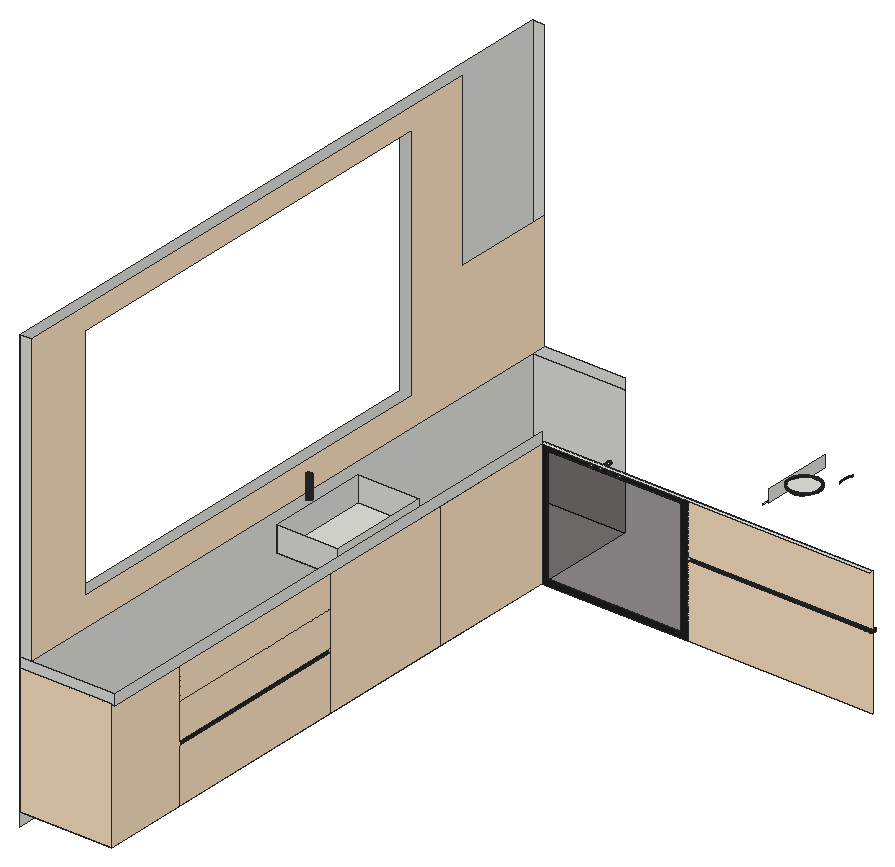
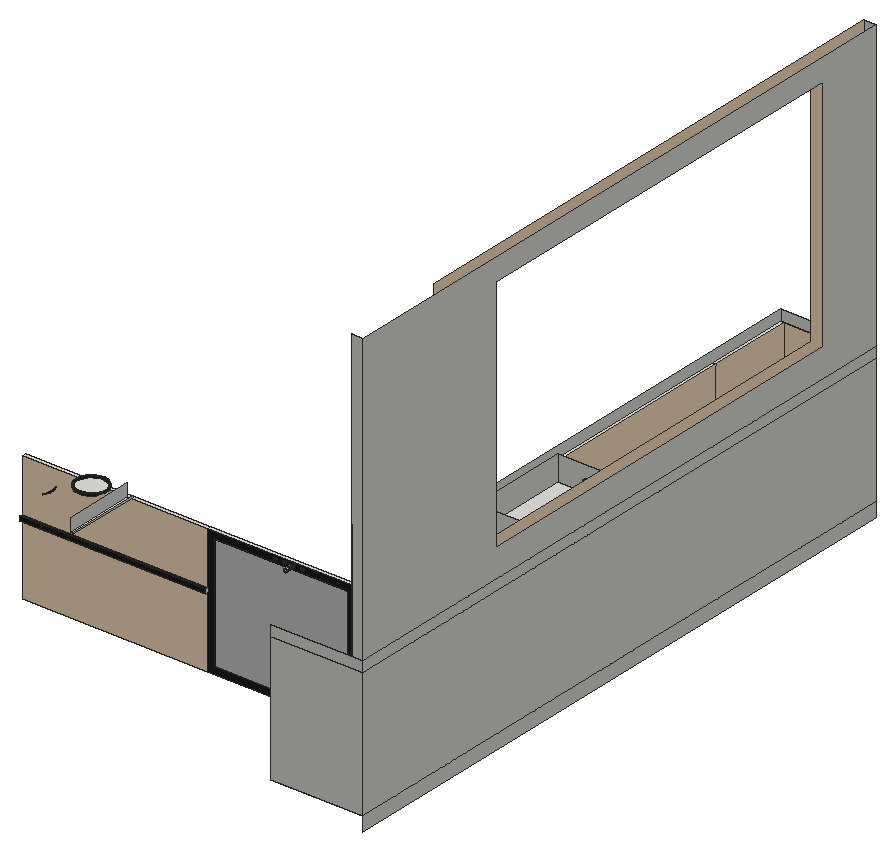
# SketchUp Ruby script. Lengths in inches.
U = 1.inch
M = Sketchup.active_model
def pt(a) = Geom::Point3d.new(a.map { |v| v * U })
def face(e, loops, mat)
  f = e.add_face(loops[0].map { |a| pt(a) })
  loops[1..].each { |l| e.add_face(l.map { |a| pt(a) }).erase! }
  f.material = f.back_material = mat if mat
  f
end
# faces: each face lists its corners as indices into pts; further lists are holes
def faces(e, pts, list, mat = nil) = list.each { |f| face(e, (f[0].is_a?(Array) ? f : [f]).map { |l| l.map { |i| pts[i] } }, mat) }
# xy, xz, yz: faces in a plane at the given z, y or x. An outline is a flat list of corners, or four numbers for a rectangle; further outlines are holes
def ring(l) = l.size == 4 ? [[l[0], l[1]], [l[2], l[1]], [l[2], l[3]], [l[0], l[3]]] : l.each_slice(2).to_a
def flat(e, list, mat, &to3) = list.each { |f| face(e, (f[0].is_a?(Array) ? f : [f]).map { |l| ring(l).map { |u, v| to3.(u, v) } }, mat) }
def xy(e, z, list, mat = nil) = flat(e, list, mat) { |x, y| [x, y, z] }
def xz(e, y, list, mat = nil) = flat(e, list, mat) { |x, z| [x, y, z] }
def yz(e, x, list, mat = nil) = flat(e, list, mat) { |y, z| [x, y, z] }
def lines(e, pts, list) = list.each { |a, b| e.add_line(pt(pts[a]), pt(pts[b])) }
# prism: a flat outline (further loops are holes) pulled along v
def prism(e, loops, v, mat = nil)
  f = face(e, loops, mat); d = Geom::Vector3d.new(v.map { |x| x * U })
  f.pushpull(f.normal.samedirection?(d) ? d.length : -d.length)
end
def box(e, o, s, mat = nil) = prism(e, [[o, [o[0] + s[0], o[1], o[2]], [o[0] + s[0], o[1] + s[1], o[2]], [o[0], o[1] + s[1], o[2]]]], [0, 0, s[2]], mat)
def at(x, y, z, deg = 0) = Geom::Transformation.translation(pt([x, y, z])) * Geom::Transformation.rotation(ORIGIN, Z_AXIS, deg.degrees)
def axes(o, x, y, z) = Geom::Transformation.new([*x, 0, *y, 0, *z, 0, *pt(o).to_a, 1])
def part(name) = M.definitions.add(name)
# library, detail: a bought-in or finely detailed component or shape, given as its bounding box
def library(name, o, s) = part(name).tap { |d| box(d.entities, o, s) }
def detail(e, o, s) = box(e.add_group.entities, o, s)
def put(e, d, t, mat = nil) = e.add_instance(d, t).tap { |i| i.material = mat if mat }
def group(e, t, mat = nil) = e.add_group.tap { |g| g.transformation = t; g.material = mat if mat }.entities
root = M.entities
M.materials.add("[0012_Bisque]").color = [255, 228, 196]
M.materials.add("[Color M00]").color = [255, 255, 255]
M.materials.add("[Color M08]").color = [30, 30, 30]
M.materials.add("[Translucent Glass Dark Green]").color = [11, 0, 5]
M.materials["[Translucent Glass Dark Green]"].alpha = 0.5
xy(root,0,[[0,2.74,25.8125,182.74]])
xy(root,15.1875,[[25.0625,26.49,25.8125,79.68]],"[Color M08]")
xy(root,16.375,[[25.0625,26.49,25.8125,79.68]],"[Color M08]")
xy(root,20.125,[[66.75,153.74,118.875,154.62]],"[Color M08]")
xy(root,21.25,[[66.75,153.74,118.875,154.62]],"[Color M08]")
xy(root,32.0625,[[7.17,83.87,24.36,112.5]])
xy(root,36,[[25.8125,2.74,26.71,26.49],[25.8125,26.49,26.71,79.68],[25.8125,79.68,26.71,118],[25.8125,118,26.71,153.74],[26.71,152.62,66.75,153.74],
  [66.75,152.62,118.875,153.74]])
xy(root,39,[[0,2.74,3.25,182.74],[5.34,96.75,5.13,96.8,4.95,96.91,4.79,97.05,4.68,97.23,4.62,97.4375,4.62,97.65,4.67,97.85,4.77,98.04,4.91,98.19,5.1,98.31,5.3,98.36,5.51,98.37,5.72,98.32,5.9,98.22,6.06,98.07,6.17,97.89,6.23,97.6875,6.23,97.48,6.18,97.27,6.08,97.08,5.93,96.93,5.75,96.82,5.55,96.76]])
xy(root,39.4375,[[84.98,158.42,85.73,178.23]])
xy(root,42.875,[[90.73,160.4,91.76,160.46,92.74,160.79,93.6,161.37,94.28,162.14,94.74,163.07,94.94,164.08,94.875,165.11,94.54,166.09,93.97,166.95,93.19,167.63,92.27,168.09,91.26,168.29,90.22,168.23,89.25,167.9,88.39,167.32,87.7,166.55,87.25,165.62,87.04,164.61,87.11,163.58,87.44,162.6,88.01,161.74,88.79,161.06,89.71,160.6]])
xy(root,42.875,[[[90.7,160.04,89.6,160.26,88.59,160.76,87.74,161.51,87.12,162.44,86.76,163.51,86.6875,164.63,86.91,165.74,87.41,166.75,88.15,167.59,89.09,168.22,90.16,168.58,91.28,168.65,92.38,168.43,93.39,167.93,94.24,167.18,94.86,166.25,95.22,165.18,95.29,164.06,95.07,162.95,94.57,161.94,93.83,161.1,92.89,160.47,91.83,160.11],[90.73,160.4,91.76,160.46,92.74,160.79,93.6,161.37,94.28,162.14,94.74,163.07,94.94,164.08,94.875,165.11,94.54,166.09,93.97,166.95,93.19,167.63,92.27,168.09,91.26,168.29,90.22,168.23,89.25,167.9,88.39,167.32,87.7,166.55,87.25,165.62,87.04,164.61,87.11,163.58,87.44,162.6,88.01,161.74,88.79,161.06,89.71,160.6]]],"[Color M08]")
xy(root,43.3125,[[[90.7,160.04,91.83,160.11,92.89,160.47,93.83,161.1,94.57,161.94,95.07,162.95,95.29,164.06,95.22,165.18,94.86,166.25,94.24,167.18,93.39,167.93,92.38,168.43,91.28,168.65,90.16,168.58,89.09,168.22,88.15,167.59,87.41,166.75,86.91,165.74,86.6875,164.63,86.76,163.51,87.12,162.44,87.74,161.51,88.59,160.76,89.6,160.26],[90.73,160.4,89.71,160.6,88.79,161.06,88.01,161.74,87.44,162.6,87.11,163.58,87.04,164.61,87.25,165.62,87.7,166.55,88.39,167.32,89.25,167.9,90.22,168.23,91.26,168.29,92.27,168.09,93.19,167.63,93.97,166.95,94.54,166.09,94.875,165.11,94.94,164.08,94.74,163.07,94.28,162.14,93.6,161.37,92.74,160.79,91.76,160.46]]],"[Color M08]")
xz(root,2.74,[[0,36,26.71,39],[0,39,3.25,120]])
xz(root,2.74,[[0,0,25.8125,36]],"[0012_Bisque]")
xz(root,26.49,[[25.0625,15.1875,25.8125,16.375]])
xz(root,79.68,[[25.0625,15.1875,25.8125,16.375]])
xz(root,83.87,[[7.17,32.0625,24.36,39]])
xz(root,112.5,[[7.17,32.0625,24.36,39]])
xz(root,153.24,[[40.09,34.75,40.2,34.76,40.31,34.81,40.4,34.88,40.47,34.97,40.51,35.07,40.53,35.1875,40.51,35.3,40.47,35.41,40.4,35.5,40.31,35.57,40.2,35.61,40.09,35.625,39.98,35.61,39.87,35.57,39.78,35.5,39.71,35.41,39.67,35.3,39.65,35.1875,39.67,35.07,39.71,34.97,39.78,34.88,39.87,34.81,39.98,34.76],[42.72,34.75,42.83,34.76,42.94,34.81,43.03,34.88,43.1,34.97,43.14,35.07,43.15,35.1875,43.14,35.3,43.1,35.41,43.03,35.5,42.94,35.57,42.83,35.61,42.72,35.625,42.6,35.61,42.5,35.57,42.41,35.5,42.34,35.41,42.29,35.3,42.28,35.1875,42.29,35.07,42.34,34.97,42.41,34.88,42.5,34.81,42.6,34.76],[45.28,34.75,45.39,34.76,45.5,34.81,45.59,34.88,45.66,34.97,45.7,35.07,45.72,35.1875,45.7,35.3,45.66,35.41,45.59,35.5,45.5,35.57,45.39,35.61,45.28,35.625,45.17,35.61,45.06,35.57,44.97,35.5,44.9,35.41,44.86,35.3,44.84,35.1875,44.86,35.07,44.9,34.97,44.97,34.88,45.06,34.81,45.17,34.76],[47.97,34.75,48.08,34.76,48.19,34.81,48.28,34.88,48.35,34.97,48.39,35.07,48.4,35.1875,48.39,35.3,48.35,35.41,48.28,35.5,48.19,35.57,48.08,35.61,47.97,35.625,47.85,35.61,47.75,35.57,47.66,35.5,47.59,35.41,47.54,35.3,47.53,35.1875,47.54,35.07,47.59,34.97,47.66,34.88,47.75,34.81,47.85,34.76]],"[Color M00]")
xz(root,153.74,[[66.75,0,118.875,20.125],[66.75,21.25,118.875,36]],"[0012_Bisque]")
xz(root,153.74,[[40.09,34.75,39.98,34.76,39.87,34.81,39.78,34.88,39.71,34.97,39.67,35.07,39.65,35.1875,39.67,35.3,39.71,35.41,39.78,35.5,39.87,35.57,39.98,35.61,40.09,35.625,40.2,35.61,40.31,35.57,40.4,35.5,40.47,35.41,40.51,35.3,40.53,35.1875,40.51,35.07,40.47,34.97,40.4,34.88,40.31,34.81,40.2,34.76],[42.72,34.75,42.6,34.76,42.5,34.81,42.41,34.88,42.34,34.97,42.29,35.07,42.28,35.1875,42.29,35.3,42.34,35.41,42.41,35.5,42.5,35.57,42.6,35.61,42.72,35.625,42.83,35.61,42.94,35.57,43.03,35.5,43.1,35.41,43.14,35.3,43.15,35.1875,43.14,35.07,43.1,34.97,43.03,34.88,42.94,34.81,42.83,34.76],[45.28,34.75,45.17,34.76,45.06,34.81,44.97,34.88,44.9,34.97,44.86,35.07,44.84,35.1875,44.86,35.3,44.9,35.41,44.97,35.5,45.06,35.57,45.17,35.61,45.28,35.625,45.39,35.61,45.5,35.57,45.59,35.5,45.66,35.41,45.7,35.3,45.72,35.1875,45.7,35.07,45.66,34.97,45.59,34.88,45.5,34.81,45.39,34.76],[47.97,34.75,47.85,34.76,47.75,34.81,47.66,34.88,47.59,34.97,47.54,35.07,47.53,35.1875,47.54,35.3,47.59,35.41,47.66,35.5,47.75,35.57,47.85,35.61,47.97,35.625,48.08,35.61,48.19,35.57,48.28,35.5,48.35,35.41,48.39,35.3,48.4,35.1875,48.39,35.07,48.35,34.97,48.28,34.88,48.19,34.81,48.08,34.76]],"[Color M00]")
xz(root,153.74,[[[25.8125,0,66.75,36],[27.6,1.79,64.96,34.21],[40.09,34.75,39.98,34.76,39.87,34.81,39.78,34.88,39.71,34.97,39.67,35.07,39.65,35.1875,39.67,35.3,39.71,35.41,39.78,35.5,39.87,35.57,39.98,35.61,40.09,35.625,40.2,35.61,40.31,35.57,40.4,35.5,40.47,35.41,40.51,35.3,40.53,35.1875,40.51,35.07,40.47,34.97,40.4,34.88,40.31,34.81,40.2,34.76],[42.72,34.75,42.6,34.76,42.5,34.81,42.41,34.88,42.34,34.97,42.29,35.07,42.28,35.1875,42.29,35.3,42.34,35.41,42.41,35.5,42.5,35.57,42.6,35.61,42.72,35.625,42.83,35.61,42.94,35.57,43.03,35.5,43.1,35.41,43.14,35.3,43.15,35.1875,43.14,35.07,43.1,34.97,43.03,34.88,42.94,34.81,42.83,34.76],[45.28,34.75,45.17,34.76,45.06,34.81,44.97,34.88,44.9,34.97,44.86,35.07,44.84,35.1875,44.86,35.3,44.9,35.41,44.97,35.5,45.06,35.57,45.17,35.61,45.28,35.625,45.39,35.61,45.5,35.57,45.59,35.5,45.66,35.41,45.7,35.3,45.72,35.1875,45.7,35.07,45.66,34.97,45.59,34.88,45.5,34.81,45.39,34.76],[47.97,34.75,47.85,34.76,47.75,34.81,47.66,34.88,47.59,34.97,47.54,35.07,47.53,35.1875,47.54,35.3,47.59,35.41,47.66,35.5,47.75,35.57,47.85,35.61,47.97,35.625,48.08,35.61,48.19,35.57,48.28,35.5,48.35,35.41,48.39,35.3,48.4,35.1875,48.39,35.07,48.35,34.97,48.28,34.88,48.19,34.81,48.08,34.76]]],"[Color M08]")
xz(root,153.74,[[27.6,1.79,64.96,34.21]],"[Translucent Glass Dark Green]")
xz(root,154.62,[[66.75,20.125,118.875,21.25]],"[Color M08]")
xz(root,156.55,[[42.72,34.75,42.6,34.76,42.5,34.81,42.41,34.88,42.34,34.97,42.29,35.07,42.28,35.1875,42.29,35.3,42.34,35.41,42.41,35.5,42.5,35.57,42.6,35.61,42.72,35.625,42.83,35.61,42.94,35.57,43.03,35.5,43.1,35.41,43.14,35.3,43.15,35.1875,43.14,35.07,43.1,34.97,43.03,34.88,42.94,34.81,42.83,34.76]],"[Color M00]")
xz(root,182.74,[[0,0,25.8125,36],[0,36,25.8125,39],[0,39,3.25,120]])
yz(root,0,[[2.74,-4,182.74,0],[2.74,0,182.74,36],[2.74,36,182.74,39],[[2.74,39,182.74,120],[21.33,47.1,136.27,113.85]]])
yz(root,3.25,[[[2.74,39,182.74,39,182.74,72,153.74,72,153.74,120,2.74,120],[21.33,47.1,136.27,113.85]]],"[0012_Bisque]")
yz(root,4.62,[[97.4375,39,97.65,45.17]])
yz(root,6.23,[[97.48,39,97.6875,44.93]])
yz(root,7.17,[[83.87,32.0625,112.5,39]])
yz(root,24.36,[[83.87,32.0625,112.5,39]])
yz(root,25.0625,[[26.49,15.1875,79.68,16.375]],"[Color M08]")
yz(root,25.8125,[[2.74,0,26.49,36],[26.49,0,79.68,15.1875],[79.68,0,118,36],[118,0,153.74,36],[26.49,16.375,79.68,26.125],
  [26.49,26.125,79.68,36]],"[0012_Bisque]")
yz(root,26.71,[[2.74,36,152.62,39]])
yz(root,66.75,[[153.74,20.125,154.62,21.25]])
yz(root,84.98,[[157.35,39,178.23,39.4375]])
yz(root,85.73,[[158.42,39.4375,178.23,42.875]])
p = [[39.98,153.74,34.76],[40.09,153.74,34.75],[40.09,153.24,34.75],[39.98,153.24,34.76],[40.2,153.74,34.76],[40.2,153.24,34.76],
  [42.6,153.74,34.76],[42.72,153.74,34.75],[42.72,153.24,34.75],[42.6,153.24,34.76],[42.83,153.74,34.76],[42.83,153.24,34.76],
  [45.17,153.74,34.76],[45.28,153.74,34.75],[45.28,153.24,34.75],[45.17,153.24,34.76],[45.39,153.74,34.76],[45.39,153.24,34.76],
  [47.85,153.74,34.76],[47.97,153.74,34.75],[47.97,153.24,34.75],[47.85,153.24,34.76],[48.08,153.74,34.76],[48.08,153.24,34.76],
  [42.6,156.55,34.76],[42.72,156.55,34.75],[42.83,156.55,34.76],[39.78,153.74,34.88],[39.87,153.74,34.81],[39.87,153.24,34.81],
  [39.78,153.24,34.88],[40.31,153.74,34.81],[40.31,153.24,34.81],[40.4,153.74,34.88],[40.4,153.24,34.88],[42.41,153.74,34.88],
  [42.5,153.74,34.81],[42.5,153.24,34.81],[42.41,153.24,34.88],[42.94,153.74,34.81],[42.94,153.24,34.81],[43.03,153.74,34.88],
  [43.03,153.24,34.88],[44.97,153.74,34.88],[45.06,153.74,34.81],[45.06,153.24,34.81],[44.97,153.24,34.88],[45.5,153.74,34.81],
  [45.5,153.24,34.81],[45.59,153.74,34.88],[45.59,153.24,34.88],[47.66,153.74,34.88],[47.75,153.74,34.81],[47.75,153.24,34.81],
  [47.66,153.24,34.88],[48.19,153.74,34.81],[48.19,153.24,34.81],[48.28,153.74,34.88],[48.28,153.24,34.88],[42.41,156.55,34.88],
  [42.5,156.55,34.81],[42.94,156.55,34.81],[43.03,156.55,34.88],[39.71,153.74,34.97],[39.71,153.24,34.97],[40.47,153.74,34.97],
  [40.47,153.24,34.97],[42.34,153.74,34.97],[42.34,153.24,34.97],[43.1,153.74,34.97],[43.1,153.24,34.97],[44.9,153.74,34.97],
  [44.9,153.24,34.97],[45.66,153.74,34.97],[45.66,153.24,34.97],[47.59,153.74,34.97],[47.59,153.24,34.97],[48.35,153.74,34.97],
  [48.35,153.24,34.97],[42.34,156.55,34.97],[43.1,156.55,34.97],[39.67,153.74,35.07],[39.67,153.24,35.07],[40.51,153.74,35.07],
  [40.51,153.24,35.07],[42.29,153.74,35.07],[42.29,153.24,35.07],[43.14,153.74,35.07],[43.14,153.24,35.07],[44.86,153.74,35.07],
  [44.86,153.24,35.07],[45.7,153.74,35.07],[45.7,153.24,35.07],[47.54,153.74,35.07],[47.54,153.24,35.07],[48.39,153.74,35.07],
  [48.39,153.24,35.07],[42.29,156.55,35.07],[43.14,156.55,35.07],[39.65,153.74,35.1875],[39.65,153.24,35.1875],[40.53,153.74,35.1875],
  [40.53,153.24,35.1875],[42.28,153.74,35.1875],[42.28,153.24,35.1875],[43.15,153.74,35.1875],[43.15,153.24,35.1875],[44.84,153.74,35.1875],
  [44.84,153.24,35.1875],[45.72,153.74,35.1875],[45.72,153.24,35.1875],[47.53,153.74,35.1875],[47.53,153.24,35.1875],[48.4,153.74,35.1875],
  [48.4,153.24,35.1875],[42.28,156.55,35.1875],[43.15,156.55,35.1875],[39.67,153.74,35.3],[39.67,153.24,35.3],[40.51,153.74,35.3],
  [40.51,153.24,35.3],[42.29,153.74,35.3],[42.29,153.24,35.3],[43.14,153.74,35.3],[43.14,153.24,35.3],[44.86,153.74,35.3],
  [44.86,153.24,35.3],[45.7,153.74,35.3],[45.7,153.24,35.3],[47.54,153.74,35.3],[47.54,153.24,35.3],[48.39,153.74,35.3],
  [48.39,153.24,35.3],[42.29,156.55,35.3],[43.14,156.55,35.3],[39.71,153.74,35.41],[39.71,153.24,35.41],[40.47,153.74,35.41],
  [40.47,153.24,35.41],[42.34,153.74,35.41],[42.34,153.24,35.41],[43.1,153.74,35.41],[43.1,153.24,35.41],[44.9,153.74,35.41],
  [44.9,153.24,35.41],[45.66,153.74,35.41],[45.66,153.24,35.41],[47.59,153.74,35.41],[47.59,153.24,35.41],[48.35,153.74,35.41],
  [48.35,153.24,35.41],[42.34,156.55,35.41],[43.1,156.55,35.41],[39.78,153.74,35.5],[39.78,153.24,35.5],[40.4,153.74,35.5],
  [40.4,153.24,35.5],[42.41,153.74,35.5],[42.41,153.24,35.5],[43.03,153.74,35.5],[43.03,153.24,35.5],[44.97,153.74,35.5],
  [44.97,153.24,35.5],[45.59,153.74,35.5],[45.59,153.24,35.5],[47.66,153.74,35.5],[47.66,153.24,35.5],[48.28,153.74,35.5],
  [48.28,153.24,35.5],[42.41,156.55,35.5],[43.03,156.55,35.5],[39.87,153.74,35.57],[39.87,153.24,35.57],[40.31,153.74,35.57],
  [40.31,153.24,35.57],[42.5,153.74,35.57],[42.5,153.24,35.57],[42.94,153.74,35.57],[42.94,153.24,35.57],[45.06,153.74,35.57],
  [45.06,153.24,35.57],[45.5,153.74,35.57],[45.5,153.24,35.57],[47.75,153.74,35.57],[47.75,153.24,35.57],[48.19,153.74,35.57],
  [48.19,153.24,35.57],[42.5,156.55,35.57],[42.94,156.55,35.57],[39.98,153.74,35.61],[39.98,153.24,35.61],[40.09,153.74,35.625],
  [40.09,153.24,35.625],[40.2,153.74,35.61],[40.2,153.24,35.61],[42.6,153.74,35.61],[42.6,153.24,35.61],[42.72,153.74,35.625],
  [42.72,153.24,35.625],[42.83,153.74,35.61],[42.83,153.24,35.61],[45.17,153.74,35.61],[45.17,153.24,35.61],[45.28,153.74,35.625],
  [45.28,153.24,35.625],[45.39,153.74,35.61],[45.39,153.24,35.61],[47.85,153.74,35.61],[47.85,153.24,35.61],[47.97,153.74,35.625],
  [47.97,153.24,35.625],[48.08,153.74,35.61],[48.08,153.24,35.61],[42.6,156.55,35.61],[42.72,156.55,35.625],[42.83,156.55,35.61],
  [4.95,96.91,39],[5.13,96.8,39],[5.13,96.8,45.1],[4.95,96.91,45.125],[5.34,96.75,39],[5.34,96.75,45.07],
  [5.55,96.76,39],[5.55,96.76,45.03],[5.75,96.82,39],[5.75,96.82,45],[5.93,96.93,39],[5.93,96.93,44.98],
  [4.79,97.05,39],[4.79,97.05,45.15],[6.08,97.08,39],[6.08,97.08,44.95],[6.08,97.08,44.96],[6.02,97.02,44.96],
  [4.68,97.23,39],[4.68,97.23,45.16],[6.18,97.27,39],[6.18,97.27,44.94],[4.62,97.4375,39],[4.62,97.4375,45.17],
  [6.23,97.48,39],[6.23,97.48,44.93],[4.67,97.85,39],[4.62,97.65,39],[4.62,97.65,45.17],[4.67,97.85,45.16],
  [6.23,97.6875,39],[6.17,97.89,39],[6.17,97.89,44.94],[6.23,97.6875,44.93],[4.77,98.04,39],[4.77,98.04,45.15],
  [6.06,98.07,39],[6.06,98.07,44.95],[6.06,98.07,44.96],[4.91,98.19,39],[4.91,98.19,45.13],[5.9,98.22,39],
  [5.9,98.22,44.98],[6.02,98.11,44.96],[5.1,98.31,39],[5.1,98.31,45.1],[5.72,98.32,39],[5.72,98.32,45.01],
  [5.3,98.36,39],[5.3,98.36,45.07],[5.51,98.37,39],[5.51,98.37,45.04],[89.6,160.26,42.875],[90.7,160.04,42.875],
  [90.7,160.04,43.3125],[89.6,160.26,43.3125],[91.83,160.11,42.875],[91.83,160.11,43.3125],[92.89,160.47,42.875],[92.89,160.47,43.3125],
  [88.59,160.76,42.875],[88.59,160.76,43.3125],[90.73,160.4,42.875],[89.71,160.6,42.875],[89.71,160.6,43.3125],[90.73,160.4,43.3125],
  [91.76,160.46,42.875],[91.76,160.46,43.3125],[92.74,160.79,42.875],[92.74,160.79,43.3125],[93.83,161.1,42.875],[93.83,161.1,43.3125],
  [88.79,161.06,42.875],[88.79,161.06,43.3125],[87.74,161.51,42.875],[87.74,161.51,43.3125],[93.6,161.37,42.875],[93.6,161.37,43.3125],
  [88.01,161.74,42.875],[88.01,161.74,43.3125],[94.57,161.94,42.875],[94.57,161.94,43.3125],[94.28,162.14,42.875],[94.28,162.14,43.3125],
  [87.12,162.44,42.875],[87.12,162.44,43.3125],[87.44,162.6,42.875],[87.44,162.6,43.3125],[95.07,162.95,42.875],[95.07,162.95,43.3125],
  [94.74,163.07,42.875],[94.74,163.07,43.3125],[86.76,163.51,42.875],[86.76,163.51,43.3125],[87.11,163.58,42.875],[87.11,163.58,43.3125],
  [95.29,164.06,42.875],[95.29,164.06,43.3125],[94.94,164.08,42.875],[94.94,164.08,43.3125],[86.6875,164.63,42.875],[86.6875,164.63,43.3125],
  [87.04,164.61,42.875],[87.04,164.61,43.3125],[94.875,165.11,42.875],[94.875,165.11,43.3125],[95.22,165.18,42.875],[95.22,165.18,43.3125],
  [86.91,165.74,42.875],[86.91,165.74,43.3125],[87.25,165.62,42.875],[87.25,165.62,43.3125],[94.54,166.09,42.875],[94.54,166.09,43.3125],
  [94.86,166.25,42.875],[94.86,166.25,43.3125],[87.7,166.55,42.875],[87.7,166.55,43.3125],[87.41,166.75,42.875],[87.41,166.75,43.3125],
  [93.97,166.95,42.875],[93.97,166.95,43.3125],[94.24,167.18,42.875],[94.24,167.18,43.3125],[88.39,167.32,42.875],[88.39,167.32,43.3125],
  [88.15,167.59,42.875],[88.15,167.59,43.3125],[93.19,167.63,42.875],[93.19,167.63,43.3125],[93.39,167.93,42.875],[93.39,167.93,43.3125],
  [89.25,167.9,42.875],[89.25,167.9,43.3125],[89.09,168.22,42.875],[89.09,168.22,43.3125],[92.27,168.09,42.875],[92.27,168.09,43.3125],
  [90.22,168.23,42.875],[90.22,168.23,43.3125],[92.38,168.43,42.875],[92.38,168.43,43.3125],[91.26,168.29,42.875],[91.26,168.29,43.3125],
  [90.16,168.58,42.875],[90.16,168.58,43.3125],[91.28,168.65,42.875],[91.28,168.65,43.3125],[96.16,170.97,42.875],[96.52,169.9,42.875],
  [96.52,169.9,43.3125],[96.16,170.97,43.3125],[96.09,172.09,42.875],[96.09,172.09,43.3125],[96.31,173.2,42.875],[96.31,173.2,43.3125],
  [96.81,174.21,42.875],[96.81,174.21,43.3125],[5.36,97.58,39],[5.36,97.58,45.0625]]
faces(root,p,[[0,1,2,3],[1,4,5,2],[6,7,8,9],[7,10,11,8],[12,13,14,15],[13,16,17,14],[18,19,20,21],[19,22,23,20],
  [7,6,24,25],[10,7,25,26],[27,28,29,30],[28,0,3,29],[4,31,32,5],[31,33,34,32],[35,36,37,38],[36,6,9,37],
  [10,39,40,11],[39,41,42,40],[43,44,45,46],[44,12,15,45],[16,47,48,17],[47,49,50,48],[51,52,53,54],[52,18,21,53],
  [22,55,56,23],[55,57,58,56],[36,35,59,60],[6,36,60,24],[39,10,26,61],[41,39,61,62],[63,27,30,64],[33,65,66,34],
  [67,35,38,68],[41,69,70,42],[71,43,46,72],[49,73,74,50],[75,51,54,76],[57,77,78,58],[35,67,79,59],[69,41,62,80],
  [81,63,64,82],[65,83,84,66],[85,67,68,86],[69,87,88,70],[89,71,72,90],[73,91,92,74],[93,75,76,94],[77,95,96,78],
  [67,85,97,79],[87,69,80,98],[99,81,82,100],[83,101,102,84],[103,85,86,104],[87,105,106,88],[107,89,90,108],[91,109,110,92],
  [111,93,94,112],[95,113,114,96],[85,103,115,97],[105,87,98,116],[117,99,100,118],[101,119,120,102],[121,103,104,122],[105,123,124,106],
  [125,107,108,126],[109,127,128,110],[129,111,112,130],[113,131,132,114],[103,121,133,115],[123,105,116,134],[135,117,118,136],[119,137,138,120],
  [139,121,122,140],[123,141,142,124],[143,125,126,144],[127,145,146,128],[147,129,130,148],[131,149,150,132],[121,139,151,133],[141,123,134,152],
  [153,135,136,154],[137,155,156,138],[157,139,140,158],[141,159,160,142],[161,143,144,162],[145,163,164,146],[165,147,148,166],[149,167,168,150],
  [139,157,169,151],[159,141,152,170],[171,153,154,172],[155,173,174,156],[175,157,158,176],[159,177,178,160],[179,161,162,180],[163,181,182,164],
  [183,165,166,184],[167,185,186,168],[157,175,187,169],[177,159,170,188],[189,171,172,190],[191,189,190,192],[193,191,192,194],[173,193,194,174],
  [195,175,176,196],[197,195,196,198],[199,197,198,200],[177,199,200,178],[201,179,180,202],[203,201,202,204],[205,203,204,206],[181,205,206,182],
  [207,183,184,208],[209,207,208,210],[211,209,210,212],[185,211,212,186],[175,195,213,187],[195,197,214,213],[197,199,215,214],[199,177,188,215]],"[Color M00]")
faces(root,p,[[216,217,218,219],[217,220,221,218],[220,222,223,221],[222,224,225,223],[224,226,227,225],[228,216,219,229],[226,230,231,232,233,227],[234,228,229,235],
  [230,236,237,232,231],[238,234,235,239],[236,240,241,237],[242,243,244,245],[246,247,248,249],[250,242,245,251],[247,252,253,254,248],[255,250,251,256],
  [252,257,258,259,254,253],[260,255,256,261],[257,262,263,258],[264,260,261,265],[262,266,267,263],[266,264,265,267]])
faces(root,p,[[268,269,270,271],[269,272,273,270],[272,274,275,273],[276,268,271,277],[278,279,280,281],[282,278,281,283],[284,282,283,285],[274,286,287,275],
  [279,288,289,280],[290,276,277,291],[292,284,285,293],[288,294,295,289],[286,296,297,287],[298,292,293,299],[300,290,291,301],[294,302,303,295],
  [296,304,305,297],[306,298,299,307],[308,300,301,309],[302,310,311,303],[304,312,313,305],[314,306,307,315],[316,308,309,317],[310,318,319,311],
  [320,314,315,321],[312,322,323,313],[324,316,317,325],[318,326,327,319],[328,320,321,329],[322,330,331,323],[326,332,333,327],[334,324,325,335],
  [336,328,329,337],[330,338,339,331],[332,340,341,333],[342,334,335,343],[344,336,337,345],[338,346,347,339],[340,348,349,341],[350,342,343,351],
  [352,344,345,353],[348,354,355,349],[346,356,357,347],[358,352,353,359],[360,350,351,361],[354,358,359,355],[356,362,363,357],[362,360,361,363],
  [364,365,366,367],[368,364,367,369],[370,368,369,371],[372,370,371,373]],"[Color M08]")
lines(root,p,[[374,375]])
